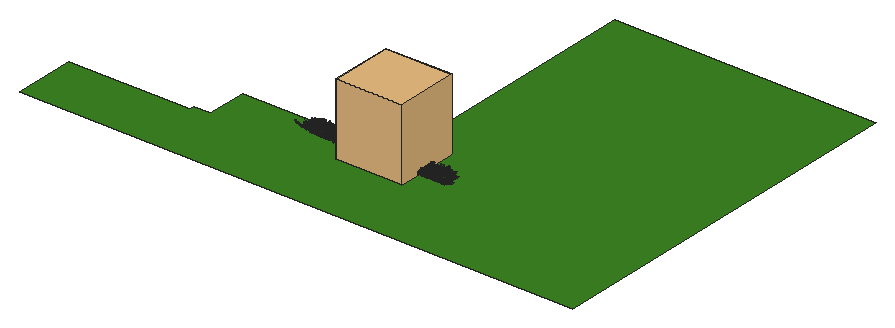
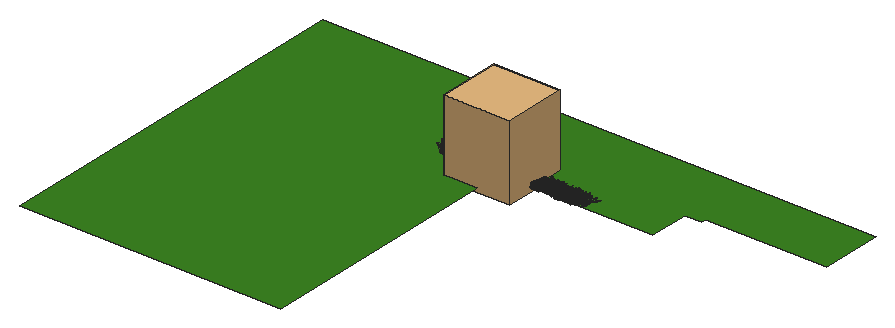
# SketchUp Ruby script. Lengths in inches.
U = 1.inch
M = Sketchup.active_model
def pt(a) = Geom::Point3d.new(a.map { |v| v * U })
def face(e, loops, mat)
  f = e.add_face(loops[0].map { |a| pt(a) })
  loops[1..].each { |l| e.add_face(l.map { |a| pt(a) }).erase! }
  f.material = f.back_material = mat if mat
  f
end
# faces: each face lists its corners as indices into pts; further lists are holes
def faces(e, pts, list, mat = nil) = list.each { |f| face(e, (f[0].is_a?(Array) ? f : [f]).map { |l| l.map { |i| pts[i] } }, mat) }
# xy, xz, yz: faces in a plane at the given z, y or x. An outline is a flat list of corners, or four numbers for a rectangle; further outlines are holes
def ring(l) = l.size == 4 ? [[l[0], l[1]], [l[2], l[1]], [l[2], l[3]], [l[0], l[3]]] : l.each_slice(2).to_a
def flat(e, list, mat, &to3) = list.each { |f| face(e, (f[0].is_a?(Array) ? f : [f]).map { |l| ring(l).map { |u, v| to3.(u, v) } }, mat) }
def xy(e, z, list, mat = nil) = flat(e, list, mat) { |x, y| [x, y, z] }
def xz(e, y, list, mat = nil) = flat(e, list, mat) { |x, z| [x, y, z] }
def yz(e, x, list, mat = nil) = flat(e, list, mat) { |y, z| [x, y, z] }
def lines(e, pts, list) = list.each { |a, b| e.add_line(pt(pts[a]), pt(pts[b])) }
# prism: a flat outline (further loops are holes) pulled along v
def prism(e, loops, v, mat = nil)
  f = face(e, loops, mat); d = Geom::Vector3d.new(v.map { |x| x * U })
  f.pushpull(f.normal.samedirection?(d) ? d.length : -d.length)
end
def box(e, o, s, mat = nil) = prism(e, [[o, [o[0] + s[0], o[1], o[2]], [o[0] + s[0], o[1] + s[1], o[2]], [o[0], o[1] + s[1], o[2]]]], [0, 0, s[2]], mat)
def at(x, y, z, deg = 0) = Geom::Transformation.translation(pt([x, y, z])) * Geom::Transformation.rotation(ORIGIN, Z_AXIS, deg.degrees)
def axes(o, x, y, z) = Geom::Transformation.new([*x, 0, *y, 0, *z, 0, *pt(o).to_a, 1])
def part(name) = M.definitions.add(name)
# library, detail: a bought-in or finely detailed component or shape, given as its bounding box
def library(name, o, s) = part(name).tap { |d| box(d.entities, o, s) }
def detail(e, o, s) = box(e.add_group.entities, o, s)
def put(e, d, t, mat = nil) = e.add_instance(d, t).tap { |i| i.material = mat if mat }
def group(e, t, mat = nil) = e.add_group.tap { |g| g.transformation = t; g.material = mat if mat }.entities
root = M.entities
M.materials.add("Material82").color = [68, 110, 58]
M.materials.add("Material83").color = [48, 90, 38]
M.materials.add("Material84").color = [68, 110, 48]
M.materials.add("Material85").color = [48, 90, 48]
M.materials.add("Material86").color = [58, 110, 58]
M.materials.add("Material87").color = [58, 90, 38]
M.materials.add("Material88").color = [68, 100, 58]
M.materials.add("Material89").color = [48, 100, 38]
M.materials.add("[Color M01]").color = [60, 133, 34]
c1 = part("grass00")
p = [[-0.6875,0.15,0],[-0.56,0.08,5.52],[-0.04,0.03,2.76],[0.48,-0.02,0],[0.35,-0.02,5.52],[-0.1,-0.14,5.52],
  [-0.12,0.65,8.37],[-0.42,0.65,8.37]]
faces(c1.entities,p,[[0,1,2,3],[3,2,4],[1,5,2],[5,4,2],[1,6,5],[4,5,6],[7,6,1]])
c2 = part("Group16\#1")
put(c2.entities,c1,axes([1.44,-0.61,-0.01],[0.05352,0.12609,0],[-0.10704,0.04543,0.07239],[0.06664,-0.02828,0.11628]),"Material85")
put(c2.entities,c1,axes([0.76,-0.15,-0.01],[0.04676,0.24062,0],[-0.23162,0.04501,0.06642],[0.0652,-0.01267,0.23595]),"Material82")
put(c2.entities,c1,axes([0.79,0.01,-0.01],[-0.00606,0.34651,0],[-0.34381,-0.00602,0.0432],[0.04319,0.00076,0.34386]))
put(c2.entities,c1,axes([1,0.23,-0.01],[-0.07192,0.31144,0],[-0.28722,-0.06632,0.1236],[0.12043,0.02781,0.29478]),"Material84")
put(c2.entities,c1,axes([1.66,0.77,-0.01],[-0.13828,0.29651,0],[-0.21551,-0.1005,0.22471],[0.20365,0.09498,0.23779]),"Material89")
put(c2.entities,c1,axes([0.6875,0.52,-0.01],[-0.18126,0.24051,0],[-0.22746,-0.17142,0.09788],[0.07817,0.05891,0.28481]),"Material84")
put(c2.entities,c1,axes([0.68,0.78,-0.01],[-0.215,0.18688,0],[-0.12385,-0.14248,0.21334],[0.13995,0.16101,0.18878]),"Material82")
put(c2.entities,c1,axes([0.56,1,-0.01],[-0.13756,0.07624,0],[-0.06159,-0.11112,0.0927],[0.04494,0.08108,0.12705]),"Material84")
put(c2.entities,c1,axes([0.2,0.64,-0.01],[-0.23729,0.07254,0],[-0.05711,-0.18681,0.153],[0.04473,0.14632,0.19535]),"Material89")
put(c2.entities,c1,axes([0.0625,0.72,-0.01],[-0.28874,0.02525,0],[-0.02179,-0.24916,0.14647],[0.01276,0.14591,0.25012]),"Material82")
put(c2.entities,c1,axes([-0.08,0.62,-0.01],[-0.34089,-0.04187,0],[0.03255,-0.26504,0.216],[-0.02633,0.21439,0.26703]),"Material89")
put(c2.entities,c1,axes([-0.34,0.98,-0.01],[-0.14314,-0.0493,0],[0.04397,-0.12769,0.06843],[-0.02228,0.0647,0.13505]),"Material89")
put(c2.entities,c1,axes([-0.87,1.45,-0.01],[-0.23488,-0.14114,0],[0.13761,-0.22901,0.06087],[-0.03135,0.05217,0.26717]))
put(c2.entities,c1,axes([-0.72,0.77,-0.01],[-0.14208,-0.13251,0],[0.07209,-0.0773,0.16301],[-0.11118,0.11922,0.1057]),"Material89")
put(c2.entities,c1,axes([-0.62,0.43,-0.01],[-0.14845,-0.21203,0],[0.18654,-0.13061,0.12304],[-0.10079,0.07057,0.22772]),"Material82")
put(c2.entities,c1,axes([-0.68,0.29,-0.01],[-0.13639,-0.32136,0],[0.31723,-0.13464,0.05579],[-0.05136,0.0218,0.34462]),"Material83")
put(c2.entities,c1,axes([-0.64,0.125,-0.01],[-0.0458,-0.23569,0],[0.22124,-0.043,0.08276],[-0.08124,0.01579,0.22538]),"Material86")
put(c2.entities,c1,axes([-1.6,-0.03,-0.01],[0.00576,-0.32897,0],[0.27526,0.00482,0.18018],[-0.18015,-0.00315,0.2753]),"Material84")
put(c2.entities,c1,axes([-1.36,-0.31,-0.01],[0.05718,-0.24765,0],[0.18172,0.04196,0.17267],[-0.16825,-0.03885,0.1865]),"Material89")
put(c2.entities,c1,axes([-1.54,-0.72,-0.01],[0.06537,-0.14017,0],[0.13555,0.06321,0.03939],[-0.0357,-0.01665,0.14956]))
put(c2.entities,c1,axes([-1.19,-0.9,-0.01],[0.09597,-0.12735,0],[0.11214,0.08451,0.07557],[-0.06035,-0.04548,0.14042]),"Material88")
put(c2.entities,c1,axes([-0.47,-0.54,-0.01],[0.11588,-0.10072,0],[0.0618,0.0711,0.12124],[-0.07953,-0.0915,0.0942]))
put(c2.entities,c1,axes([-0.47,-0.84,-0.01],[0.11927,-0.0661,0],[0.06603,0.11913,0.00646],[-0.00313,-0.00565,0.13621]),"Material84")
put(c2.entities,c1,axes([-0.38,-1.24,-0.01],[0.28037,-0.08571,0],[0.0618,0.20215,0.20315],[-0.05939,-0.19428,0.21139]),"Material88")
put(c2.entities,c1,axes([-0.06,-0.66,-0.01],[0.22719,-0.01987,0],[0.01247,0.14255,0.17758],[-0.01547,-0.17691,0.1431]),"Material87")
put(c2.entities,c1,axes([0.11,-0.89,-0.01],[0.14882,0.01828,0],[-0.01058,0.08611,0.12229],[0.01491,-0.12138,0.08676]),"Material85")
put(c2.entities,c1,axes([0.25,-0.72,-0.01],[0.20481,0.07053,0],[-0.06206,0.18022,0.10291],[0.03351,-0.0973,0.1906]),"Material85")
put(c2.entities,c1,axes([0.85,-1.42,-0.01],[0.16481,0.09904,0],[-0.09472,0.15762,0.05616],[0.02893,-0.04814,0.18389]),"Material84")
put(c2.entities,c1,axes([1.01,-1.09,-0.01],[0.21858,0.20385,0],[-0.17495,0.1876,0.15339],[0.10462,-0.11218,0.25652]),"Material89")
put(c2.entities,c1,axes([1.01,-0.71,-0.01],[0.08733,0.12473,0],[-0.06445,0.04512,0.13037],[0.1068,-0.07477,0.07867]),"Material85")
c3 = part("Group15\#1")
put(c3.entities,c2,at(0,0,0))
c4 = part("3darcstudiotree_grass00\#1")
put(c4.entities,c3,at(0,0,0))
c5 = library("Flora+17",[-57.52,158.6,-38.64],[66.99,62.88,77.28])
xy(root,-34.17,[[486.41,273.41,1048.66,273.41,1048.66,659.09,782.78,659.09,782.78,381.72,626.68,381.72,626.68,341.03,609.09,341.03,609.09,335.84,486.41,335.84]],"[Color M01]")
put(root,c4,axes([744.53,368.1,-34.17],[4.00543,0.63259,0],[-1.51384,1.49079,-0.05201],[-0.11143,0.10973,1.75905]))
put(root,c4,axes([786.4,368.38,-34.17],[-2.53432,-1.16731,0],[3.13366,-1.05813,-0.03189],[0.12006,-0.04054,1.53238]))
put(root,c4,axes([756.42,368.98,-34.17],[2.98326,-0.56932,0],[1.56375,1.27443,-0.0104],[0.02417,0.0197,1.43546]))
put(root,c4,axes([734.71,368.18,-34.17],[-2.79487,1.34009,0],[-3.4856,-1.13062,-0.01702],[-0.07434,-0.02411,1.91367]))
put(root,c4,axes([795.5625,368.37,-34.17],[-1.68076,1.66641,0],[-3.14491,-0.49334,-0.04072],[-0.22908,-0.03594,1.53595]))
put(root,c4,axes([772.05,368.59,-34.17],[0.66214,1.69294,0],[-3.60919,0.21955,-0.0058],[-0.03794,0.00231,1.813]))
put(root,c4,axes([822.04,368.72,-34.17],[-3.64575,-0.40954,0],[1.09452,-1.51542,-0.03955],[0.07063,-0.09779,1.95202]))
put(root,c4,axes([731.28,368.83,-34.17],[-3.63168,-0.94551,0],[2.04917,-1.22414,-0.0411],[0.11661,-0.06966,1.43569]))
put(root,c4,axes([812.58,368.6875,-34.17],[-4.50339,0.12702,0],[-0.32923,-1.8154,-0.06114],[-0.02191,-0.12082,1.73764]))
put(root,c4,axes([827.23,369.12,-34.17],[3.9368,0.32867,0],[-0.7645,1.42421,-0.03259],[-0.03941,0.07343,1.61556]))
put(root,c4,axes([799.72,369.1,-34.17],[-1.97756,-1.20873,0],[2.87461,-0.73146,-0.04434],[0.19177,-0.0488,1.31982]))
put(root,c4,axes([769.14,368.64,-34.17],[-0.80195,1.7338,0],[-4.65742,-0.33505,-0.02378],[-0.12913,-0.00929,1.95907]))
put(root,c4,axes([719.48,368.9375,-34.17],[1.69594,1.55136,0],[-4.25972,0.72425,-0.01792],[-0.06344,0.01079,1.34035]))
put(root,c4,axes([839.08,368.75,-34.17],[-0.96856,1.32293,0],[-4.17213,-0.47507,-0.01983],[-0.0846,-0.00963,1.44555]))
put(root,c4,axes([816.69,368.93,-34.17],[-4.11343,-0.37841,0],[0.77008,-1.30194,-0.01564],[0.01915,-0.03238,1.3694]))
put(root,c4,axes([713.92,368.84,-34.17],[-1.08101,1.66314,0],[-4.29936,-0.43462,-0.05431],[-0.26643,-0.02693,1.6847]))
put(root,c4,axes([730.92,369.72,-34.17],[3.51633,-0.36112,0],[0.9428,1.4278,-0.03218],[0.03818,0.05783,1.32043]))
put(root,c4,axes([761.56,369,-34.17],[-3.19418,0.83767,0],[-2.09756,-1.24397,-0.00165],[-0.00457,-0.00271,1.42237]))
put(root,c4,axes([769.48,369.79,-34.17],[4.46941,0.03034,0],[-0.07094,1.62545,-0.04862],[-0.00377,0.08633,1.39123]))
put(root,c4,axes([791.89,370.15,-34.17],[3.30112,0.44872,0],[-1.07202,1.22659,-0.01199],[-0.02088,0.02389,1.31812]))
put(root,c4,axes([782.8125,369.98,-34.17],[2.54447,1.0037,0],[-2.66541,1.05092,-0.04694],[-0.19938,0.07861,1.69685]))
put(root,c4,axes([747.85,369.8,-34.17],[-2.46131,1.0799,0],[-2.93079,-1.03891,-0.05045],[-0.18868,-0.06689,1.48531]))
put(root,c4,axes([796.21,370.08,-34.17],[1.71949,1.25443,0],[-3.5766,0.76249,-0.00296],[-0.01327,0.00283,1.55057]))
put(root,c4,axes([706.45,369.73,-34.17],[-4.32286,0.64319,0],[-1.64772,-1.72238,-0.03096],[-0.05617,-0.05872,1.79846]))
put(root,c4,axes([828.66,369.84,-34.17],[-0.85979,1.68043,0],[-3.51636,-0.27982,-0.00527],[-0.03686,-0.00293,1.91768]))
put(root,c4,axes([740.2,370.32,-34.17],[-1.06768,-1.28552,0],[4.42505,-0.5716,-0.01545],[0.0652,-0.00842,1.54954]))
put(root,c4,axes([756.53,370.78,-34.17],[1.44921,-1.37247,0],[3.47001,0.56986,-0.04485],[0.23379,0.03839,1.59096]))
put(root,c4,axes([802.8,371.03,-34.17],[2.98286,-1.36319,0],[2.94856,1.00345,-0.04774],[0.23651,0.08049,1.91023]))
put(root,c4,axes([780.96,370.375,-34.17],[-4.5512,0.12899,0],[-0.29843,-1.6376,-0.01837],[-0.00647,-0.03552,1.53349]))
put(root,c4,axes([713.8,370.79,-34.17],[2.63123,0.92373,0],[-2.85346,1.26414,-0.03405],[-0.11674,0.05172,1.65877]))
put(root,c4,axes([833.44,371.19,-34.17],[2.31859,-1.24057,0],[3.7429,1.08799,-0.00987],[0.04342,0.01262,1.9048]))
put(root,c4,axes([806.48,370.77,-34.17],[3.00883,1.26771,0],[-3.0504,1.12602,-0.05678],[-0.17699,0.06533,1.337]))
put(root,c4,axes([818.72,371.19,-34.17],[2.02967,-1.41693,0],[3.62772,0.8082,-0.05349],[0.29346,0.06538,1.96798]))
put(root,c4,axes([763.89,371.26,-34.17],[3.59827,-1.20315,0],[2.55541,1.18863,-0.04452],[0.1901,0.08842,1.95574]))
put(root,c4,axes([771.83,370.5,-34.17],[-2.59269,1.36416,0],[-3.43206,-1.0145,-0.01976],[-0.08545,-0.02526,1.7373]))
put(root,c4,axes([749.65,370.72,-34.17],[0.38941,1.44392,0],[-4.06327,0.17043,-0.05804],[-0.26328,0.01104,1.39706]))
put(root,c4,axes([736.38,371.14,-34.17],[-0.85342,-1.31702,0],[3.52172,-0.35493,-0.03508],[0.23842,-0.02403,1.91126]))
put(root,c4,axes([824.04,371.09,-34.17],[-1.26608,-1.23533,0],[3.94424,-0.62872,-0.05241],[0.25484,-0.04062,1.67241]))
put(root,c4,axes([719.13,371.22,-34.17],[2.49471,1.02577,0],[-2.71621,1.02741,-0.02632],[-0.13149,0.04974,1.95302]))
put(root,c4,axes([812.26,371.13,-34.17],[-2.51394,1.47726,0],[-3.35133,-0.88701,-0.03945],[-0.17377,-0.04599,1.6047]))
put(root,c4,axes([724.27,371.15,-34.17],[-3.75575,0.69708,0],[-1.71963,-1.441,-0.0027],[-0.006,-0.00502,1.57765]))
put(root,c4,axes([767.14,372.17,-34.17],[4.01141,-0.57098,0],[1.38004,1.50792,-0.00463],[0.00922,0.01007,1.7876]))
put(root,c4,axes([783.03,372.35,-34.17],[1.0408,-1.70786,0],[3.59221,0.34047,-0.00397],[0.02558,0.00242,1.83602]))
put(root,c4,axes([835.61,371.99,-34.17],[1.31466,1.33352,0],[-4.27103,0.65487,-0.01993],[-0.10773,0.01652,1.99239]))
put(root,c4,axes([771.59,372.54,-34.17],[4.23995,-0.14734,0],[0.39715,1.77755,-0.00682],[0.00263,0.01179,1.49182]))
put(root,c4,axes([755.43,371.97,-34.17],[-3.94041,-0.17555,0],[0.52244,-1.82386,-0.03054],[0.01805,-0.06303,1.83699]))
put(root,c4,axes([718.57,372,-34.17],[-3.80907,0.85988,0],[-1.7501,-1.20575,-0.03218],[-0.10036,-0.06914,1.65786]))
put(root,c4,axes([830.21,372.31,-34.17],[3.99583,0.96728,0],[-1.88023,1.20803,-0.0354],[-0.13352,0.08578,1.94218]))
put(root,c4,axes([802.04,372.2,-34.17],[1.07934,1.49635,0],[-4.41478,0.49528,-0.01266],[-0.0607,0.00681,1.71446]))
put(root,c4,axes([747.49,372.04,-34.17],[-1.53161,1.39817,0],[-3.93212,-0.66992,-0.05011],[-0.24211,-0.04125,1.6899]))
put(root,c4,axes([710.71,372.73,-34.17],[0.46065,-1.85098,0],[4.3401,0.16799,-0.05803],[0.23131,0.00895,1.30918]))
put(root,c4,axes([727.48,372.1,-34.17],[-2.75394,0.84395,0],[-2.86283,-1.45294,-0.03993],[-0.13572,-0.06888,1.9372]))
put(root,c4,axes([790.64,372.39,-34.17],[-3.99444,-0.7583,0],[1.47781,-1.21073,-0.01121],[0.03612,-0.02959,1.89718]))
put(root,c4,axes([708.27,372.38,-34.17],[-2.97002,-0.61033,0],[1.81963,-1.37718,-0.0201],[0.04091,-0.03096,1.30027]))
put(root,c4,axes([822.6,372.29,-34.17],[0.15484,1.66312,0],[-4.06716,0.05889,-0.05084],[-0.28361,0.00411,1.70302]))
put(root,c4,axes([762.28,372.22,-34.17],[-1.75851,1.2095,0],[-3.69968,-0.83659,-0.01882],[-0.09945,-0.02249,1.94745]))
put(root,c4,axes([807.96,372.6875,-34.17],[1.72171,1.1824,0],[-3.73214,0.84521,-0.0451],[-0.23455,0.05312,1.93445]))
put(root,c4,axes([818.71,373.33,-34.17],[0.19619,-1.71635,0],[3.31321,0.0589,-0.03915],[0.30696,0.00546,1.95085]))
put(root,c4,axes([752.82,372.79,-34.17],[-0.47592,1.56401,0],[-3.26389,-0.15447,-0.01529],[-0.10295,-0.00487,1.67142]))
put(root,c4,axes([725.28,372.97,-34.17],[-0.69376,1.57067,0],[-3.29157,-0.22612,-0.03897],[-0.27242,-0.01871,1.77692]))
put(root,c4,axes([738.4,372.93,-34.17],[-3.02696,1.26281,0],[-2.89442,-1.07905,-0.01805],[-0.07526,-0.02806,1.71251]))
put(root,c4,axes([796.3,373.11,-34.17],[-0.66988,1.5554,0],[-4.19746,-0.28116,-0.06003],[-0.34231,-0.02293,1.84592]))
put(root,c4,axes([736.17,373.2,-34.17],[-1.89755,1.14164,0],[-2.79539,-0.72263,-0.04],[-0.1948,-0.05036,1.45882]))
put(root,c4,axes([779.9,373.36,-34.17],[-1.94069,1.13311,0],[-3.87728,-1.03282,-0.01862],[-0.08293,-0.02209,1.88514]))
put(root,c4,axes([807.77,374.12,-34.17],[1.1935,-1.34336,0],[4.3339,0.59885,-0.02001],[0.09738,0.01346,1.77455]))
put(root,c4,axes([811.51,373.36,-34.17],[-2.50228,1.03927,0],[-3.36492,-1.26006,-0.01749],[-0.0653,-0.02445,1.7911]))
put(root,c4,axes([708.51,374.14,-34.17],[3.05945,-1.08948,0],[2.66485,1.16389,-0.04418],[0.16678,0.07284,1.67893]))
put(root,c4,axes([734.66,374.46,-34.17],[4.28763,0.74332,0],[-1.60811,1.44267,-0.02572],[-0.05083,0.0456,1.47108]))
put(root,c4,axes([821.55,374.74,-34.17],[3.2454,-0.59836,0],[1.90263,1.60498,-0.04906],[0.1129,0.09524,1.82977]))
put(root,c4,axes([750.47,374.5,-34.17],[-3.62624,-0.35306,0],[1.02554,-1.63824,-0.03453],[0.0374,-0.05975,1.44935]))
put(root,c4,axes([740.4,374.81,-34.17],[4.10391,0.70985,0],[-1.57565,1.41679,-0.04488],[-0.12117,0.10895,1.97665]))
put(root,c4,axes([773.66,374.5,-34.17],[-4.00947,-0.30727,0],[0.87061,-1.76683,-0.00093],[0.00074,-0.0015,1.42207]))
put(root,c4,axes([802.83,375.04,-34.17],[3.36205,-0.0702,0],[0.18049,1.34442,-0.02933],[0.01197,0.08919,1.97542]))
put(root,c4,axes([838.49,374.89,-34.17],[-3.24576,-0.77305,0],[1.70346,-1.11239,-0.04514],[0.15554,-0.10157,1.64638]))
put(root,c4,axes([811.27,374.53,-34.17],[-2.83529,0.94791,0],[-2.49489,-1.16063,-0.0209],[-0.0692,-0.03219,1.48072]))
put(root,c4,axes([768.02,375.3,-34.17],[2.86215,-0.69885,0],[2.15737,1.37418,-0.03178],[0.09016,0.05743,1.65559]))
put(root,c4,axes([818.1,374.86,-34.17],[-4.36996,-0.43983,0],[0.81337,-1.25688,-0.00096],[0.00152,-0.00235,1.58162]))
put(root,c4,axes([743.89,375.43,-34.17],[3.05285,-0.84724,0],[2.57962,1.44566,-0.04926],[0.16288,0.09128,1.93034]))
put(root,c4,axes([782.54,375,-34.17],[2.0306,1.51402,0],[-3.86929,0.80712,-0.01033],[-0.04249,0.00886,1.52631]))
put(root,c4,axes([727.26,374.91,-34.17],[-4.22095,0.29279,0],[-0.61258,-1.3735,-0.03096],[-0.02808,-0.06297,1.38775]))
put(root,c4,axes([724.24,375.08,-34.17],[-3.27374,-0.87824,0],[2.36689,-1.37221,-0.01911],[0.04526,-0.02624,1.32815]))
put(root,c4,axes([716.5,375.66,-34.17],[1.2731,-1.20941,0],[3.44603,0.56418,-0.03248],[0.17294,0.02831,1.61223]))
put(root,c4,axes([763.1,375.47,-34.17],[2.55345,1.05656,0],[-3.3838,1.27189,-0.0237],[-0.06613,0.02486,1.35093]))
put(root,c4,axes([710.6875,375.25,-34.17],[1.1355,1.36945,0],[-3.88951,0.50159,-0.05705],[-0.27012,0.03483,1.52794]))
put(root,c4,axes([791.77,375.57,-34.17],[4.32541,0.68003,0],[-1.26335,1.24977,-0.02018],[-0.04043,0.04,1.38364]))
put(root,c4,axes([758.34,375.13,-34.17],[-2.26024,1.36544,0],[-3.77789,-0.97262,-0.02867],[-0.12669,-0.03262,1.78429]))
put(root,c4,axes([828.89,375.37,-34.17],[-1.11192,1.29739,0],[-3.39488,-0.45252,-0.04196],[-0.24016,-0.03201,1.62262]))
put(root,c4,axes([796.42,375.57,-34.17],[-3.14118,-0.50543,0],[1.51948,-1.46871,-0.03312],[0.08056,-0.07787,1.94116]))
put(root,c4,axes([835.72,375.41,-34.17],[-3.94382,0.34286,0],[-0.79478,-1.42188,-0.01188],[-0.01845,-0.03301,1.99665]))
put(root,c4,axes([780.38,375.51,-34.17],[-4.08544,0.78173,0],[-2.02978,-1.64985,-0.06144],[-0.10479,-0.08517,1.3618]))
put(root,c4,axes([817.9,376.3,-34.17],[0.47621,-1.80202,0],[3.38439,0.1391,-0.02929],[0.17813,0.00732,1.55926]))
put(root,c4,axes([735.87,376.72,-34.17],[3.68176,-0.08889,0],[0.28452,1.83295,-0.0507],[0.01477,0.09515,1.66388]))
put(root,c4,axes([833.08,376.84,-34.17],[4.51376,-0.38644,0],[0.93116,1.69158,-0.03342],[0.04124,0.07493,1.91382]))
put(root,c4,axes([731.14,376.99,-34.17],[3.55776,-0.23199,0],[0.75341,1.79699,-0.01648],[0.0118,0.02815,1.51991]))
put(root,c4,axes([738.7,376.23,-34.17],[-2.26269,0.97698,0],[-3.46591,-1.24844,-0.00484],[-0.01583,-0.0057,1.55938]))
put(root,c4,axes([724.13,376.53,-34.17],[-0.84248,1.5623,0],[-4.12413,-0.34589,-0.02719],[-0.15102,-0.01267,1.79436]))
put(root,c4,axes([766.09,376.78,-34.17],[1.45585,1.40356,0],[-4.29762,0.69331,-0.06498],[-0.33385,0.05386,1.93183]))
put(root,c4,axes([771.79,377.44,-34.17],[2.50638,-0.90958,0],[2.96207,1.26944,-0.00074],[0.00258,0.00111,1.68668]))
put(root,c4,axes([800.89,377.34,-34.17],[2.93855,-0.93601,0],[2.3882,1.16609,-0.03491],[0.14245,0.06955,1.84986]))
put(root,c4,axes([788.69,377.17,-34.17],[3.70843,0.7821,0],[-1.67561,1.2357,-0.00407],[-0.01146,0.00845,1.59208]))
put(root,c4,axes([711.5,377.26,-34.17],[-2.75759,-1.29294,0],[3.16062,-1.04842,-0.04595],[0.19898,-0.066,1.75181]))
put(root,c4,axes([810.82,377.08,-34.17],[-3.51736,-0.62046,0],[1.43276,-1.26324,-0.00732],[0.0191,-0.01684,1.68082]))
put(root,c5,at(807.92,187.19,0))
put(root,c4,axes([827.2,377.58,-34.17],[1.17526,-1.64902,0],[4.03097,0.44682,-0.04021],[0.21409,0.02373,1.73573]))
put(root,c4,axes([705.78,377.43,-34.17],[3.8564,0.72862,0],[-1.8534,1.52567,-0.04599],[-0.08438,0.06946,1.36526]))
put(root,c4,axes([758.48,377.73,-34.17],[2.63553,-1.14097,0],[3.49929,1.25715,-0.04921],[0.17097,0.06142,1.66765]))
put(root,c4,axes([778.9375,377.46,-34.17],[-2.13357,-1.0721,0],[3.45076,-1.06807,-0.04646],[0.2021,-0.06255,1.81816]))
put(root,c4,axes([824.9375,377.69,-34.17],[3.33693,-0.09981,0],[0.31842,1.6558,-0.06006],[0.02203,0.11454,1.53056]))
put(root,c4,axes([795.37,377.86,-34.17],[1.17971,-1.62892,0],[3.63954,0.40996,-0.01145],[0.05532,0.00623,1.42532]))
put(root,c4,axes([744.21,377.29,-34.17],[-4.27172,-0.34301,0],[0.88739,-1.71879,-0.03896],[0.04123,-0.07985,1.76791]))
put(root,c4,axes([764.34,377.48,-34.17],[1.4209,1.26091,0],[-3.92098,0.6872,-0.00487],[-0.02309,0.00405,1.66894]))
put(root,c4,axes([805.68,377.52,-34.17],[-2.4369,-0.91248,0],[2.76412,-1.14811,-0.01822],[0.07791,-0.03236,1.86907]))
put(root,c4,axes([751.28,377.49,-34.17],[-4.07234,0.0884,0],[-0.21728,-1.55677,-0.00024],[-0.00008,-0.0006,1.85086]))
put(root,c4,axes([716.06,377.59,-34.17],[-0.67685,1.82709,0],[-3.63349,-0.20935,-0.03578],[-0.17247,-0.00994,1.34076]))
put(root,c4,axes([783.59,377.67,-34.17],[-4.28311,0.42951,0],[-0.86146,-1.33607,-0.01716],[-0.03026,-0.04692,1.87475]))
put(root,c4,axes([785.86,378.42,-34.17],[3.93391,0.38635,0],[-0.92741,1.4687,-0.04825],[-0.05916,0.09369,1.45973]))
put(root,c4,axes([797.61,378.82,-34.17],[1.5424,-1.39232,0],[4.02917,0.6942,-0.02716],[0.11079,0.01909,1.46706]))
put(root,c4,axes([806.33,378.64,-34.17],[-3.14575,-1.33265,0],[2.56413,-0.94137,-0.04944],[0.22162,-0.08136,1.60821]))
put(root,c4,axes([823.05,378.89,-34.17],[3.16271,-0.89527,0],[1.91794,1.05379,-0.02763],[0.08663,0.0476,1.3256]))
put(root,c4,axes([719.48,378.85,-34.17],[4.09109,-0.59758,0],[1.20224,1.2801,-0.03178],[0.07676,0.08173,1.80429]))
put(root,c4,axes([769.27,378.84,-34.17],[0.03648,-1.32003,0],[3.51668,0.01511,-0.01263],[0.08154,0.00035,1.70174]))
put(root,c4,axes([788.41,378.8,-34.17],[2.84603,0.80034,0],[-2.3016,1.27293,-0.03635],[-0.10022,0.05543,1.41103]))
put(root,c4,axes([775.125,379.15,-34.17],[0.45602,-1.75469,0],[4.51141,0.18235,-0.06373],[0.28019,0.01133,1.50237]))
put(root,c4,axes([813.9,378.88,-34.17],[2.37182,1.09167,0],[-3.5393,1.19596,-0.05975],[-0.18065,0.06104,1.3909]))
put(root,c4,axes([745.25,379.19,-34.17],[4.21739,-0.2744,0],[0.59088,1.41243,-0.03976],[0.04192,0.1002,1.7619]))
put(root,c4,axes([728.36,378.73,-34.17],[-4.11616,0.08361,0],[-0.21641,-1.65704,-0.00589],[-0.00131,-0.01,1.35922]))
put(root,c4,axes([706.69,379,-34.17],[1.39303,1.55232,0],[-3.39855,0.47433,-0.0171],[-0.11021,0.01538,1.84743]))
put(root,c4,axes([817.7,379.62,-34.17],[1.48234,-1.44208,0],[4.35208,0.69577,-0.03495],[0.16928,0.02706,1.83937]))
put(root,c4,axes([779.51,378.91,-34.17],[-3.86986,1.0079,0],[-2.20275,-1.31539,-0.01955],[-0.05283,-0.03155,1.46911]))
put(root,c4,axes([833.34,379.78,-34.17],[2.23867,-1.3669,0],[3.69886,0.94218,-0.0579],[0.27243,0.06939,1.84885]))
put(root,c4,axes([829.39,379.52,-34.17],[-1.90503,-1.23869,0],[3.27066,-0.78232,-0.01057],[0.0584,-0.01397,1.85267]))
put(root,c4,axes([711.03,379.89,-34.17],[2.18609,-1.17283,0],[3.5885,1.04029,-0.0227],[0.08817,0.02556,1.60931]))
put(root,c4,axes([739.87,379.79,-34.17],[4.1241,0.10126,0],[-0.23149,1.46627,-0.04181],[-0.01816,0.11501,1.95138]))
put(root,c4,axes([755.54,379.4,-34.17],[-3.62534,0.37466,0],[-0.93047,-1.40031,-0.00505],[-0.0081,-0.01218,1.74136]))
put(root,c4,axes([735.99,379.48,-34.17],[-4.14933,0.35699,0],[-0.86081,-1.55612,-0.03649],[-0.04634,-0.08377,1.80375]))
put(root,c4,axes([763.8125,379.87,-34.17],[-1.44336,-1.26835,0],[3.91991,-0.69378,-0.01184],[0.05292,-0.00937,1.57815]))
put(root,c4,axes([723.26,379.66,-34.17],[-3.20067,0.8851,0],[-2.09814,-1.18003,-0.04222],[-0.15558,-0.0875,1.75818]))
put(root,c4,axes([800.02,379.85,-34.17],[-2.84152,0.97731,0],[-2.62045,-1.18497,-0.0546],[-0.22213,-0.10045,1.84968]))
put(root,c4,axes([749.375,380,-34.17],[0.82539,1.5958,0],[-3.41483,0.2747,-0.03877],[-0.28197,0.02268,1.93915]))
put(root,c4,axes([761.84,380.81,-34.17],[4.36048,0.20882,0],[-0.42656,1.38529,-0.01966],[-0.01597,0.05186,1.78732]))
put(root,c4,axes([712.16,381.05,-34.17],[4.28771,-0.12133,0],[0.32919,1.80935,-0.01186],[0.00375,0.02059,1.52253]))
put(root,c4,axes([797.7,380.65,-34.17],[-2.28475,-0.97473,0],[2.77585,-1.01196,-0.01026],[0.04604,-0.01678,1.73127]))
put(root,c4,axes([827.0625,380.61,-34.17],[1.07114,1.64692,0],[-4.05863,0.41055,-0.04684],[-0.20509,0.02075,1.41954]))
put(root,c4,axes([755.8125,380.63,-34.17],[0.44153,1.60869,0],[-4.59886,0.19631,-0.03135],[-0.13775,0.00588,1.53244]))
put(root,c4,axes([791.51,380.7,-34.17],[0.72726,1.40914,0],[-3.71927,0.29854,-0.02796],[-0.18755,0.01505,1.94708]))
put(root,c4,axes([767.73,380.86,-34.17],[2.07536,1.00802,0],[-2.97078,0.95128,-0.04172],[-0.20153,0.06453,1.78477]))
put(root,c4,axes([774.79,381.11,-34.17],[-2.23262,-1.3088,0],[3.58665,-0.95157,-0.0439],[0.1738,-0.04611,1.54604]))
put(root,c4,axes([807.88,381.24,-34.17],[-2.0126,-1.62184,0],[4.11765,-0.79471,-0.06506],[0.29073,-0.05611,1.70958]))
put(root,c4,axes([800.19,380.65,-34.17],[-3.10197,1.07124,0],[-2.38472,-1.07399,-0.00238],[-0.01101,-0.00496,1.90825]))
put(root,c4,axes([817.39,380.9,-34.17],[-3.67787,-0.26396,0],[0.66039,-1.43112,-0.02729],[0.03307,-0.07167,1.8715]))
put(root,c4,axes([824.51,381.46,-34.17],[-0.88129,-1.68738,0],[3.67182,-0.29826,-0.02826],[0.15697,-0.01275,1.59374]))
put(root,c4,axes([744.19,380.95,-34.17],[-2.93173,0.8474,0],[-2.63832,-1.41962,-0.02359],[-0.06961,-0.03745,1.66971]))
put(root,c4,axes([722.17,381.68,-34.17],[-0.92548,-1.44714,0],[3.73119,-0.37112,-0.02503],[0.12441,-0.01237,1.47852]))
put(root,c4,axes([785.07,381.72,-34.17],[-1.15236,-1.67434,0],[3.65122,-0.39084,-0.0298],[0.14551,-0.01558,1.43464]))
put(root,c4,axes([834.55,381.48,-34.17],[0.85919,1.59494,0],[-3.67668,0.30804,-0.01067],[-0.0678,0.00568,1.82972]))
